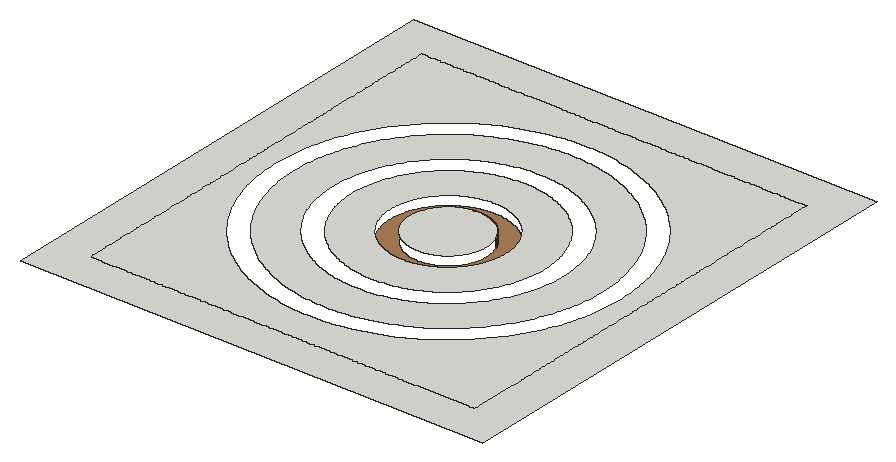
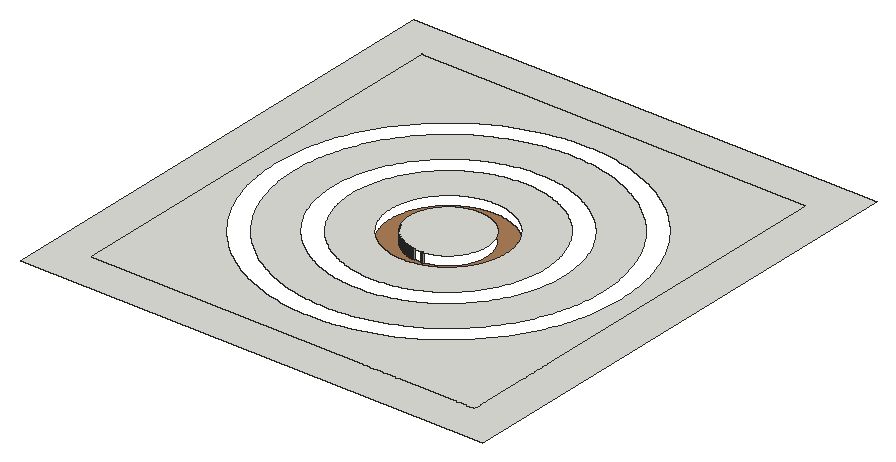
# SketchUp Ruby script. Lengths in inches.
U = 1.inch
M = Sketchup.active_model
def pt(a) = Geom::Point3d.new(a.map { |v| v * U })
def face(e, loops, mat)
  f = e.add_face(loops[0].map { |a| pt(a) })
  loops[1..].each { |l| e.add_face(l.map { |a| pt(a) }).erase! }
  f.material = f.back_material = mat if mat
  f
end
# faces: each face lists its corners as indices into pts; further lists are holes
def faces(e, pts, list, mat = nil) = list.each { |f| face(e, (f[0].is_a?(Array) ? f : [f]).map { |l| l.map { |i| pts[i] } }, mat) }
# xy, xz, yz: faces in a plane at the given z, y or x. An outline is a flat list of corners, or four numbers for a rectangle; further outlines are holes
def ring(l) = l.size == 4 ? [[l[0], l[1]], [l[2], l[1]], [l[2], l[3]], [l[0], l[3]]] : l.each_slice(2).to_a
def flat(e, list, mat, &to3) = list.each { |f| face(e, (f[0].is_a?(Array) ? f : [f]).map { |l| ring(l).map { |u, v| to3.(u, v) } }, mat) }
def xy(e, z, list, mat = nil) = flat(e, list, mat) { |x, y| [x, y, z] }
def xz(e, y, list, mat = nil) = flat(e, list, mat) { |x, z| [x, y, z] }
def yz(e, x, list, mat = nil) = flat(e, list, mat) { |y, z| [x, y, z] }
def lines(e, pts, list) = list.each { |a, b| e.add_line(pt(pts[a]), pt(pts[b])) }
# prism: a flat outline (further loops are holes) pulled along v
def prism(e, loops, v, mat = nil)
  f = face(e, loops, mat); d = Geom::Vector3d.new(v.map { |x| x * U })
  f.pushpull(f.normal.samedirection?(d) ? d.length : -d.length)
end
def box(e, o, s, mat = nil) = prism(e, [[o, [o[0] + s[0], o[1], o[2]], [o[0] + s[0], o[1] + s[1], o[2]], [o[0], o[1] + s[1], o[2]]]], [0, 0, s[2]], mat)
def at(x, y, z, deg = 0) = Geom::Transformation.translation(pt([x, y, z])) * Geom::Transformation.rotation(ORIGIN, Z_AXIS, deg.degrees)
def axes(o, x, y, z) = Geom::Transformation.new([*x, 0, *y, 0, *z, 0, *pt(o).to_a, 1])
def part(name) = M.definitions.add(name)
# library, detail: a bought-in or finely detailed component or shape, given as its bounding box
def library(name, o, s) = part(name).tap { |d| box(d.entities, o, s) }
def detail(e, o, s) = box(e.add_group.entities, o, s)
def put(e, d, t, mat = nil) = e.add_instance(d, t).tap { |i| i.material = mat if mat }
def group(e, t, mat = nil) = e.add_group.tap { |g| g.transformation = t; g.material = mat if mat }.entities
root = M.entities
M.materials.add("01 - Default1").color = [173, 128, 89]
xy(root,111.3125,[[[905.98,289.26,905.04,289.27,904.09,289.31,903.15,289.37,902.22,289.45,901.28,289.5625,900.35,289.7,899.42,289.86,898.49,290.04,897.57,290.25,896.66,290.48,895.75,290.74,894.85,291.02,893.96,291.32,893.08,291.65,892.2,292,891.34,292.37,890.48,292.76,889.64,293.18,888.8,293.62,887.98,294.08,887.17,294.5625,886.37,295.0625,885.59,295.59,884.82,296.13,884.0625,296.7,883.32,297.28,882.6,297.88,881.89,298.5,881.2,299.14,880.52,299.8,879.87,300.48,879.23,301.17,878.6,301.875,878,302.6,877.42,303.34,876.85,304.1,876.31,304.87,875.79,305.65,875.28,306.45,874.8,307.26,874.34,308.08,873.9,308.91,873.49,309.76,873.09,310.61,872.72,311.48,872.37,312.35,872.04,313.24,871.74,314.13,871.46,315.03,871.21,315.9375,870.97,316.85,870.77,317.77,870.58,318.7,870.42,319.625,870.29,320.56,870.18,321.49,870.09,322.43,870.03,323.37,869.99,324.3125,869.98,325.26,869.99,326.2,870.03,327.14,870.09,328.08,870.18,329.02,870.29,329.96,870.42,330.89,870.58,331.82,870.77,332.74,870.97,333.66,871.21,334.57,871.46,335.48,871.74,336.38,872.04,337.27,872.37,338.16,872.72,339.03,873.09,339.9,873.49,340.75,873.9,341.6,874.34,342.43,874.8,343.26,875.28,344.07,875.79,344.86,876.31,345.65,876.85,346.42,877.42,347.17,878,347.91,878.6,348.64,879.23,349.34,879.87,350.04,880.52,350.71,881.2,351.37,881.89,352.01,882.6,352.63,883.32,353.23,884.0625,353.82,884.82,354.38,885.59,354.92,886.37,355.45,887.17,355.95,887.98,356.43,888.8,356.89,889.64,357.33,890.48,357.75,891.34,358.14,892.2,358.52,893.08,358.87,893.96,359.19,894.85,359.49,895.75,359.77,896.66,360.03,897.57,360.26,898.49,360.47,899.42,360.65,900.35,360.8125,901.28,360.95,902.22,361.06,903.15,361.15,904.09,361.21,905.04,361.24,905.98,361.26,906.92,361.24,907.86,361.21,908.8,361.15,909.74,361.06,910.68,360.95,911.61,360.8125,912.54,360.65,913.46,360.47,914.38,360.26,915.3,360.03,916.2,359.77,917.1,359.49,918,359.19,918.88,358.87,919.76,358.52,920.62,358.14,921.48,357.75,922.32,357.33,923.16,356.89,923.98,356.43,924.79,355.95,925.59,355.45,926.37,354.92,927.14,354.38,927.89,353.82,928.63,353.23,929.36,352.63,930.07,352.01,930.76,351.37,931.43,350.71,932.09,350.04,932.73,349.34,933.35,348.64,933.96,347.91,934.54,347.17,935.1,346.42,935.65,345.65,936.17,344.86,936.67,344.07,937.16,343.26,937.62,342.43,938.05,341.6,938.47,340.75,938.87,339.9,939.24,339.03,939.59,338.16,939.91,337.27,940.22,336.38,940.5,335.48,940.75,334.57,940.98,333.66,941.19,332.74,941.375,331.82,941.54,330.89,941.67,329.96,941.78,329.02,941.87,328.08,941.93,327.14,941.97,326.2,941.98,325.26,941.97,324.3125,941.93,323.37,941.87,322.43,941.78,321.49,941.67,320.56,941.54,319.625,941.375,318.7,941.19,317.77,940.98,316.85,940.75,315.9375,940.5,315.03,940.22,314.13,939.91,313.24,939.59,312.35,939.24,311.48,938.87,310.61,938.47,309.76,938.05,308.91,937.62,308.08,937.16,307.26,936.67,306.45,936.17,305.65,935.65,304.87,935.1,304.1,934.54,303.34,933.96,302.6,933.35,301.875,932.73,301.17,932.09,300.48,931.43,299.8,930.76,299.14,930.07,298.5,929.36,297.88,928.63,297.28,927.89,296.7,927.14,296.13,926.37,295.59,925.59,295.0625,924.79,294.5625,923.98,294.08,923.16,293.62,922.32,293.18,921.48,292.76,920.62,292.37,919.76,292,918.88,291.65,918,291.32,917.1,291.02,916.2,290.74,915.3,290.48,914.38,290.25,913.46,290.04,912.54,289.86,911.61,289.7,910.68,289.5625,909.74,289.45,908.8,289.37,907.86,289.31,906.92,289.27],[905.35,301.26,906.61,301.26,907.23,301.29,907.86,301.33,908.49,301.39,909.11,301.46,909.73,301.55,910.35,301.66,910.97,301.78,911.58,301.92,912.19,302.07,912.8,302.24,913.4,302.43,913.99,302.63,914.58,302.85,915.16,303.08,915.74,303.33,916.3125,303.59,916.875,303.87,917.43,304.16,917.98,304.47,918.52,304.79,919.05,305.13,919.57,305.48,920.09,305.84,920.59,306.22,921.08,306.6,921.57,307.01,922.04,307.42,922.5,307.85,922.95,308.29,923.39,308.74,923.8125,309.2,924.23,309.67,924.63,310.15,925.02,310.65,925.4,311.15,925.76,311.66,926.11,312.18,926.44,312.72,926.76,313.26,927.07,313.8,927.36,314.36,927.64,314.92,927.9,315.49,928.15,316.07,928.38,316.66,928.6,317.24,928.8,317.84,928.99,318.44,929.16,319.04,929.32,319.65,929.45,320.27,929.58,320.88,929.68,321.5,929.77,322.125,929.85,322.75,929.95,324,929.97,324.63,929.98,325.26,929.97,325.88,929.95,326.51,929.9,327.14,929.85,327.76,929.77,328.39,929.68,329.01,929.58,329.63,929.45,330.25,929.32,330.86,929.16,331.47,928.99,332.07,928.8,332.67,928.6,333.27,928.38,333.86,928.15,334.44,927.9,335.02,927.64,335.59,927.36,336.15,927.07,336.71,926.76,337.26,926.44,337.8,926.11,338.33,925.76,338.85,925.4,339.36,925.02,339.87,924.63,340.36,924.23,340.84,923.8125,341.32,923.39,341.78,922.95,342.23,922.5,342.67,922.04,343.09,921.57,343.51,921.08,343.91,920.59,344.3,920.09,344.67,919.57,345.04,919.05,345.38,918.52,345.72,917.98,346.04,917.43,346.35,916.875,346.64,916.3125,346.92,915.74,347.18,915.16,347.43,914.58,347.66,913.99,347.88,913.4,348.08,912.8,348.27,912.19,348.4375,911.58,348.59,910.97,348.73,910.35,348.85,909.73,348.96,909.11,349.05,908.49,349.125,907.86,349.18,907.23,349.22,906.61,349.25,905.98,349.26,905.35,349.25,904.72,349.22,904.1,349.18,903.47,349.125,902.85,349.05,902.22,348.96,901.61,348.85,900.99,348.73,900.375,348.59,899.77,348.4375,899.16,348.27,898.5625,348.08,897.97,347.88,897.38,347.66,896.79,347.43,896.22,347.18,895.65,346.92,895.08,346.64,894.53,346.35,893.98,346.04,893.4375,345.72,892.91,345.38,892.38,345.04,891.87,344.67,891.37,344.3,890.875,343.91,890.39,343.51,889.92,343.09,889.46,342.67,889.01,342.23,888.57,341.78,888.14,341.32,887.73,340.84,887.33,340.36,886.9375,339.87,886.5625,339.36,886.2,338.85,885.85,338.33,885.52,337.8,885.19,337.26,884.89,336.71,884.59,336.15,884.32,335.59,884.05,335.02,883.57,333.86,883.36,333.27,883.15,332.67,882.97,332.07,882.8,331.47,882.64,330.86,882.5,330.25,882.38,329.63,882.27,329.01,882.18,328.39,882.11,327.76,882.05,327.14,882.01,326.51,881.99,325.88,881.98,325.26,881.99,324.63,882.01,324,882.05,323.375,882.11,322.75,882.18,322.125,882.27,321.5,882.38,320.88,882.5,320.27,882.64,319.65,882.8,319.04,882.97,318.44,883.15,317.84,883.36,317.24,883.57,316.66,883.81,316.07,884.05,315.49,884.32,314.92,884.59,314.36,884.89,313.8,885.19,313.26,885.85,312.18,886.2,311.66,886.5625,311.15,886.9375,310.65,887.33,310.15,887.73,309.67,888.14,309.2,888.57,308.74,889.01,308.29,889.46,307.85,889.92,307.42,890.39,307.01,890.875,306.6,891.37,306.22,891.87,305.84,892.38,305.48,892.91,305.13,893.4375,304.79,893.98,304.47,894.53,304.16,895.08,303.87,895.65,303.59,896.22,303.33,896.79,303.08,897.38,302.85,897.97,302.63,898.5625,302.43,899.16,302.24,899.77,302.07,900.375,301.92,900.99,301.78,901.61,301.66,902.22,301.55,902.85,301.46,903.47,301.39,904.1,301.33,904.72,301.29]]],"01 - Default1")
xy(root,117.3125,[[[761.98,172.26,1049.98,478.26],[785.98,196.26,1025.98,454.26]],[[785.98,196.26,1025.98,454.26],[905.89,217.26,908.71,217.29,911.54,217.4,914.36,217.58,917.18,217.84,919.98,218.17,922.78,218.57,925.57,219.05,928.34,219.6,931.1,220.22,933.84,220.91,936.5625,221.68,939.26,222.51,941.94,223.42,944.6,224.4,947.22,225.44,949.82,226.56,952.39,227.74,954.93,228.99,957.43,230.3,959.9,231.68,962.33,233.12,964.72,234.63,967.07,236.2,969.38,237.83,971.65,239.52,973.87,241.27,976.05,243.07,978.18,244.93,980.25,246.85,982.28,248.82,984.25,250.85,986.18,252.92,988.04,255.05,989.85,257.22,991.6,259.4375,993.3,261.7,994.93,264.01,996.5,266.36,998.02,268.75,999.46,271.18,1000.85,273.64,1002.17,276.14,1003.42,278.68,1004.6,281.24,1005.72,283.84,1006.77,286.47,1007.75,289.12,1008.66,291.79,1009.5,294.49,1010.27,297.21,1010.97,299.95,1011.6,302.71,1012.15,305.48,1012.63,308.27,1013.04,311.07,1013.38,313.875,1013.64,316.69,1013.83,319.51,1013.9375,322.34,1013.98,325.16,1013.94,327.99,1013.84,330.82,1013.65,333.64,1013.4,336.45,1013.07,339.26,1012.66,342.06,1012.1875,344.85,1011.64,347.62,1011.02,350.38,1010.32,353.12,1009.56,355.84,1008.72,358.54,1007.82,361.22,1006.84,363.87,1005.79,366.5,1004.68,369.1,1003.5,371.67,1002.25,374.2,1000.94,376.71,999.56,379.18,998.11,381.61,996.61,384,995.04,386.35,993.41,388.66,991.72,390.93,989.97,393.15,988.16,395.33,986.3,397.45,984.38,399.53,982.41,401.56,980.39,403.53,978.3125,405.45,976.19,407.32,974.02,409.13,971.8,410.88,969.53,412.58,967.23,414.21,964.88,415.78,962.49,417.29,960.06,418.74,957.59,420.125,955.09,421.44,952.56,422.7,949.99,423.88,947.39,425,944.77,426.05,942.12,427.03,939.44,427.94,936.74,428.78,934.02,429.55,931.28,430.25,928.52,430.875,925.75,431.43,922.97,431.91,920.17,432.32,917.36,432.65,914.55,432.92,911.72,433.1,908.9,433.22,906.07,433.26,903.24,433.22,900.42,433.11,897.6,432.93,894.78,432.67,891.97,432.34,889.18,431.94,886.39,431.46,883.62,430.92,880.86,430.29,878.12,429.6,875.39,428.84,872.69,428,870.02,427.09,867.36,426.12,864.74,425.07,862.14,423.96,859.57,422.78,857.03,421.53,854.53,420.21,852.06,418.83,849.63,417.39,847.24,415.88,844.88,414.31,842.57,412.68,840.31,411,838.08,409.25,835.91,407.44,833.78,405.58,831.7,403.66,829.68,401.69,827.7,399.67,825.78,397.59,823.92,395.47,822.11,393.3,820.35,391.08,818.66,388.8125,817.03,386.5,815.45,384.16,813.94,381.77,812.49,379.34,811.11,376.87,809.79,374.37,808.54,371.84,807.35,369.27,806.24,366.67,805.19,364.05,804.2,361.4,803.29,358.72,802.45,356.02,801.68,353.3,800.98,350.56,800.36,347.8,799.8,345.03,799.32,342.24,798.91,339.45,798.58,336.64,798.32,333.82,798.13,331,798.02,328.18,797.98,325.35,798.01,322.52,798.12,319.7,798.3,316.875,798.5625,314.06,798.89,311.25,799.29,308.45,799.77,305.67,800.32,302.89,800.94,300.13,801.63,297.39,802.4,294.67,803.24,291.97,804.14,289.29,805.12,286.64,806.16,284.01,807.28,281.41,808.46,278.85,809.71,276.31,811.02,273.81,812.4,271.34,813.84,268.91,815.35,266.51,816.92,264.16,818.55,261.85,820.24,259.58,821.99,257.36,823.79,255.1875,825.66,253.06,827.57,250.98,829.55,248.95,831.57,246.98,833.64,245.06,835.77,243.19,837.94,241.38,840.16,239.63,842.42,237.9375,844.73,236.3,847.08,234.73,849.47,233.22,851.9,231.77,854.36,230.39,856.86,229.07,859.4,227.82,861.97,226.63,864.5625,225.51,867.1875,224.46,869.84,223.48,872.52,222.57,875.22,221.73,877.9375,220.96,880.68,220.26,883.43,219.64,886.21,219.08,888.99,218.6,891.79,218.19,894.6,217.86,897.41,217.6,900.23,217.41,903.06,217.3]],[[905.98,229.26,903.47,229.29,900.95,229.39,898.45,229.55,895.94,229.78,893.45,230.08,890.96,230.4375,888.48,230.86,886.02,231.35,883.57,231.91,881.13,232.53,878.71,233.21,876.3125,233.95,873.93,234.76,871.58,235.63,869.24,236.5625,866.93,237.56,864.65,238.61,862.4,239.72,860.17,240.89,857.98,242.12,855.82,243.4,853.69,244.74,851.6,246.14,849.55,247.59,847.54,249.09,845.5625,250.65,843.63,252.26,841.74,253.91,839.9,255.62,838.1,257.375,836.34,259.17,834.64,261.02,832.98,262.91,831.37,264.84,829.82,266.82,828.3125,268.83,826.86,270.88,825.47,272.97,824.125,275.1,822.84,277.26,821.61,279.45,820.44,281.67,819.33,283.93,818.28,286.21,817.29,288.52,816.35,290.85,815.49,293.21,814.68,295.59,813.93,297.99,813.25,300.41,812.63,302.85,812.08,305.3,811.59,307.76,811.16,310.24,810.8,312.73,810.5,315.22,810.27,317.72,810.11,320.23,810.01,322.74,809.98,325.26,810.01,327.77,810.11,330.28,810.27,332.79,810.5,335.29,810.8,337.79,811.16,340.27,811.59,342.75,812.08,345.22,812.63,347.67,813.25,350.1,813.93,352.52,814.68,354.92,815.49,357.3,816.35,359.66,817.29,361.99,818.28,364.3,819.33,366.59,820.44,368.84,821.61,371.0625,822.84,373.26,824.125,375.42,825.47,377.54,826.86,379.63,828.3125,381.68,829.82,383.7,831.37,385.67,832.98,387.6,834.64,389.49,836.34,391.34,838.1,393.14,839.9,394.89,841.74,396.6,843.63,398.26,845.5625,399.86,847.54,401.42,849.55,402.92,851.6,404.37,853.69,405.77,855.82,407.11,857.98,408.39,860.17,409.62,862.4,410.79,864.65,411.9,866.93,412.96,869.24,413.95,871.58,414.88,873.93,415.75,876.3125,416.56,878.71,417.3,881.13,417.99,883.57,418.6,886.02,419.16,888.48,419.65,890.96,420.07,893.45,420.43,895.94,420.73,898.45,420.96,900.95,421.125,903.47,421.22,905.98,421.26,908.49,421.22,911,421.125,913.51,420.96,916.01,420.73,918.51,420.43,921,420.07,923.47,419.65,925.9375,419.16,928.39,418.6,930.83,417.99,933.24,417.3,935.64,416.56,938.02,415.75,940.38,414.88,942.72,413.95,945.03,412.96,947.31,411.9,949.5625,410.79,951.79,409.62,953.98,408.39,956.14,407.11,958.26,405.77,960.35,404.37,962.41,402.92,964.42,401.42,966.39,399.86,968.33,398.26,970.22,396.6,972.0625,394.89,973.86,393.14,975.61,391.34,977.32,389.49,978.98,387.6,980.58,385.67,982.14,383.7,983.64,381.68,985.09,379.63,986.49,377.54,987.83,375.42,989.12,373.26,990.35,371.0625,991.52,368.84,992.625,366.59,993.68,364.3,994.67,361.99,995.6,359.66,996.47,357.3,997.28,354.92,998.03,352.52,998.71,350.1,999.33,347.67,999.88,345.22,1000.37,342.75,1000.8,340.27,1001.16,337.79,1001.45,335.29,1001.68,332.79,1001.85,330.28,1001.95,327.77,1001.98,325.26,1001.95,322.74,1001.85,320.23,1001.68,317.72,1001.45,315.22,1001.16,312.73,1000.8,310.24,1000.37,307.76,999.88,305.3,999.33,302.85,998.71,300.41,998.03,297.99,997.28,295.59,996.47,293.21,995.6,290.85,994.67,288.52,993.68,286.21,992.625,283.93,991.52,281.67,990.35,279.45,989.12,277.26,987.83,275.1,986.49,272.97,985.09,270.88,983.64,268.83,982.14,266.82,980.58,264.84,978.98,262.91,977.32,261.02,975.61,259.17,973.86,257.375,972.0625,255.62,970.22,253.91,968.33,252.26,966.39,250.65,964.42,249.09,962.41,247.59,960.35,246.14,958.26,244.74,956.14,243.4,953.98,242.12,951.79,240.89,949.5625,239.72,947.31,238.61,945.03,237.56,942.72,236.5625,940.38,235.63,938.02,234.76,935.64,233.95,933.24,233.21,930.83,232.53,928.39,231.91,925.9375,231.35,923.47,230.86,921,230.4375,918.51,230.08,916.01,229.78,913.51,229.55,911,229.39,908.49,229.29],[905.98,253.26,907.86,253.28,909.75,253.35,911.63,253.48,913.5,253.65,915.375,253.87,917.24,254.14,919.1,254.46,920.95,254.83,922.79,255.25,924.61,255.71,926.43,256.22,928.23,256.78,930.01,257.39,931.78,258.04,933.53,258.74,935.26,259.48,936.98,260.27,938.67,261.1,940.33,261.98,941.98,262.9,943.6,263.87,945.19,264.87,946.76,265.92,948.3,267.01,949.81,268.13,951.29,269.3,952.74,270.51,954.16,271.75,955.54,273.03,956.89,274.34,958.21,275.69,959.49,277.08,960.73,278.5,961.93,279.95,963.1,281.43,964.23,282.9375,965.32,284.47,966.36,286.04,967.37,287.64,968.33,289.26,969.25,290.9,970.13,292.57,970.96,294.26,971.75,295.97,972.5,297.7,973.2,299.45,973.85,301.22,974.45,303.01,975.01,304.81,975.53,306.62,975.99,308.45,976.41,310.29,976.77,312.14,977.09,313.99,977.36,315.86,977.58,317.73,977.76,319.61,977.88,321.49,977.95,323.37,977.98,325.26,977.95,327.14,977.88,329.02,977.76,330.91,977.58,332.78,977.36,334.65,977.09,336.52,976.77,338.38,976.41,340.23,975.99,342.0625,975.53,343.89,975.01,345.71,974.45,347.51,973.85,349.29,973.2,351.06,972.5,352.81,971.75,354.54,970.96,356.25,970.13,357.94,969.25,359.61,968.33,361.26,967.37,362.875,966.36,364.47,965.32,366.04,964.23,367.58,963.1,369.09,961.93,370.57,960.73,372.02,959.49,373.43,958.21,374.82,956.89,376.17,955.54,377.48,954.16,378.76,952.74,380.01,951.29,381.21,949.81,382.38,948.3,383.51,946.76,384.59,945.19,385.64,943.6,386.65,941.98,387.61,940.33,388.53,938.67,389.41,936.98,390.24,935.26,391.03,933.53,391.78,931.78,392.47,930.01,393.125,928.23,393.73,926.43,394.29,924.61,394.8,922.79,395.27,920.95,395.68,919.1,396.05,917.24,396.37,915.375,396.64,913.5,396.86,911.63,397.03,909.75,397.16,907.86,397.23,905.98,397.26,904.09,397.23,902.21,397.16,900.33,397.03,898.45,396.86,896.58,396.64,894.72,396.37,892.86,396.05,891.01,395.68,889.17,395.27,887.34,394.8,885.53,394.29,883.73,393.73,881.94,393.125,880.18,392.47,878.43,391.78,876.69,391.03,874.98,390.24,873.29,389.41,871.625,388.53,869.98,387.61,868.36,386.65,866.76,385.64,865.2,384.59,863.66,383.51,862.15,382.38,860.67,381.21,859.22,380.01,857.8,378.76,856.42,377.48,855.07,376.17,853.75,374.82,852.47,373.43,851.23,372.02,850.02,370.57,848.86,369.09,847.73,367.58,846.64,366.04,845.59,364.47,844.59,362.875,843.625,361.26,842.7,359.61,841.83,357.94,840.99,356.25,840.2,354.54,839.46,352.81,838.76,351.06,838.11,349.29,837.5,347.51,836.94,345.71,836.43,343.89,835.97,342.0625,835.55,340.23,835.18,338.38,834.87,336.52,834.59,334.65,834.375,332.78,834.2,330.91,834.08,329.02,834,327.14,833.98,325.26,834,323.37,834.08,321.49,834.2,319.61,834.375,317.73,834.59,315.86,834.87,313.99,835.18,312.14,835.55,310.29,835.97,308.45,836.43,306.62,836.94,304.81,837.5,303.01,838.11,301.22,838.76,299.45,839.46,297.7,840.2,295.97,840.99,294.26,841.83,292.57,842.7,290.9,843.625,289.26,844.59,287.64,845.59,286.04,846.64,284.47,847.73,282.9375,848.86,281.43,850.02,279.95,851.23,278.5,852.47,277.08,853.75,275.69,855.07,274.34,856.42,273.03,857.8,271.75,859.22,270.51,860.67,269.3,862.15,268.13,863.66,267.01,865.2,265.92,866.76,264.87,868.36,263.87,869.98,262.9,871.625,261.98,873.29,261.1,874.98,260.27,876.69,259.48,878.43,258.74,880.18,258.04,881.94,257.39,883.73,256.78,885.53,256.22,887.34,255.71,889.17,255.25,891.01,254.83,892.86,254.46,894.72,254.14,896.58,253.87,898.45,253.65,900.33,253.48,902.21,253.35,904.09,253.28]],[[905.98,265.26,904.41,265.28,902.84,265.34,901.27,265.44,899.71,265.58,898.15,265.77,896.59,265.99,895.04,266.26,893.5,266.57,891.97,266.91,890.45,267.3,888.9375,267.73,887.4375,268.19,885.95,268.7,884.48,269.24,883.02,269.82,881.57,270.44,880.15,271.1,878.74,271.8,877.35,272.53,875.98,273.29,874.63,274.1,873.3,274.9375,871.99,275.81,870.71,276.72,869.45,277.66,868.22,278.63,867.01,279.63,865.83,280.67,864.68,281.73,863.55,282.83,862.46,283.95,861.39,285.11,860.35,286.29,859.35,287.5,858.38,288.73,857.4375,289.99,856.53,291.27,855.66,292.58,854.82,293.91,854.02,295.26,853.25,296.625,852.52,298.02,851.82,299.43,851.17,300.85,850.55,302.3,849.96,303.75,849.42,305.23,848.92,306.72,848.45,308.22,848.02,309.73,847.64,311.25,847.29,312.78,846.98,314.32,846.72,315.87,846.49,317.42,846.31,318.98,846.16,320.55,846.0625,322.12,846,323.6875,845.98,325.26,846,326.83,846.0625,328.4,846.16,329.96,846.31,331.53,846.49,333.09,846.72,334.64,846.98,336.19,847.29,337.73,847.64,339.26,848.02,340.79,848.45,342.3,848.92,343.8,849.42,345.28,849.96,346.76,850.55,348.22,851.17,349.66,851.82,351.09,852.52,352.5,853.25,353.89,854.02,355.26,854.82,356.61,855.66,357.93,856.53,359.24,857.4375,360.52,858.38,361.78,859.35,363.02,860.35,364.22,861.39,365.4,862.46,366.56,863.55,367.68,864.68,368.78,865.83,369.84,867.01,370.88,868.22,371.88,869.45,372.86,870.71,373.8,871.99,374.7,873.3,375.58,874.63,376.41,875.98,377.22,877.35,377.99,878.74,378.72,880.15,379.41,881.57,380.07,883.02,380.6875,884.48,381.27,885.95,381.81,887.4375,382.32,888.9375,382.79,890.45,383.21,891.97,383.6,893.5,383.95,895.04,384.25,896.59,384.52,898.15,384.74,899.71,384.93,901.27,385.07,902.84,385.17,904.41,385.24,905.98,385.26,907.55,385.24,909.12,385.17,910.6875,385.07,912.25,384.93,913.81,384.74,915.36,384.52,916.91,384.25,918.45,383.95,919.99,383.6,921.51,383.21,923.02,382.79,924.52,382.32,926.01,381.81,927.48,381.27,928.94,380.6875,930.38,380.07,931.81,379.41,933.22,378.72,934.61,377.99,935.98,377.22,937.33,376.41,938.66,375.58,939.96,374.7,941.25,373.8,942.5,372.86,943.74,371.88,944.95,370.88,946.125,369.84,947.28,368.78,948.41,367.68,949.5,366.56,950.57,365.4,951.6,364.22,952.61,363.02,953.58,361.78,954.52,360.52,955.43,359.24,956.3,357.93,957.14,356.61,957.94,355.26,958.71,353.89,959.4375,352.5,960.13,351.09,960.79,349.66,961.41,348.22,961.99,346.76,962.54,345.28,963.04,343.8,963.51,342.3,963.93,340.79,964.32,339.26,964.67,337.73,964.97,336.19,965.24,334.64,965.47,333.09,965.65,331.53,965.79,329.96,965.9,328.4,965.96,326.83,965.98,325.26,965.96,323.6875,965.9,322.12,965.79,320.55,965.65,318.98,965.47,317.42,965.24,315.87,964.97,314.32,964.67,312.78,964.32,311.25,963.93,309.73,963.51,308.22,963.04,306.72,962.54,305.23,961.99,303.75,961.41,302.3,960.79,300.85,960.13,299.43,959.4375,298.02,958.71,296.625,957.94,295.26,957.14,293.91,956.3,292.58,955.43,291.27,954.52,289.99,953.58,288.73,952.61,287.5,951.6,286.29,950.57,285.11,949.5,283.95,948.41,282.83,947.28,281.73,946.125,280.67,944.95,279.63,943.74,278.63,942.5,277.66,941.25,276.72,939.96,275.81,938.66,274.9375,937.33,274.1,935.98,273.29,934.61,272.53,933.22,271.8,931.81,271.1,930.38,270.44,928.94,269.82,927.48,269.24,926.01,268.7,924.52,268.19,923.02,267.73,921.51,267.3,919.99,266.91,918.45,266.57,916.91,266.26,915.36,265.99,913.81,265.77,912.25,265.58,910.6875,265.44,909.12,265.34,907.55,265.28],[905.98,289.26,906.92,289.27,907.86,289.31,908.8,289.37,909.74,289.45,910.68,289.5625,911.61,289.7,912.54,289.86,913.46,290.04,914.38,290.25,915.3,290.48,916.2,290.74,917.1,291.02,918,291.32,918.88,291.65,919.76,292,920.62,292.37,921.48,292.76,922.32,293.18,923.16,293.62,923.98,294.08,924.79,294.5625,925.59,295.0625,926.37,295.59,927.14,296.13,927.89,296.7,928.63,297.28,929.36,297.88,930.07,298.5,930.76,299.14,931.43,299.8,932.09,300.48,932.73,301.17,933.35,301.875,933.96,302.6,934.54,303.34,935.1,304.1,935.65,304.87,936.17,305.65,936.67,306.45,937.16,307.26,937.62,308.08,938.05,308.91,938.47,309.76,938.87,310.61,939.24,311.48,939.59,312.35,939.91,313.24,940.22,314.13,940.5,315.03,940.75,315.9375,940.98,316.85,941.19,317.77,941.375,318.7,941.54,319.625,941.67,320.56,941.78,321.49,941.87,322.43,941.93,323.37,941.97,324.3125,941.98,325.26,941.97,326.2,941.93,327.14,941.87,328.08,941.78,329.02,941.67,329.96,941.54,330.89,941.375,331.82,941.19,332.74,940.98,333.66,940.75,334.57,940.5,335.48,940.22,336.38,939.91,337.27,939.59,338.16,939.24,339.03,938.87,339.9,938.47,340.75,938.05,341.6,937.62,342.43,937.16,343.26,936.67,344.07,936.17,344.86,935.65,345.65,935.1,346.42,934.54,347.17,933.96,347.91,933.35,348.64,932.73,349.34,932.09,350.04,931.43,350.71,930.76,351.37,930.07,352.01,929.36,352.63,928.63,353.23,927.89,353.82,927.14,354.38,926.37,354.92,925.59,355.45,924.79,355.95,923.98,356.43,923.16,356.89,922.32,357.33,921.48,357.75,920.62,358.14,919.76,358.52,918.88,358.87,918,359.19,917.1,359.49,916.2,359.77,915.3,360.03,914.38,360.26,913.46,360.47,912.54,360.65,911.61,360.8125,910.68,360.95,909.74,361.06,908.8,361.15,907.86,361.21,906.92,361.24,905.98,361.26,905.04,361.24,904.09,361.21,903.15,361.15,902.22,361.06,901.28,360.95,900.35,360.8125,899.42,360.65,898.49,360.47,897.57,360.26,896.66,360.03,895.75,359.77,894.85,359.49,893.96,359.19,893.08,358.87,892.2,358.52,891.34,358.14,890.48,357.75,889.64,357.33,888.8,356.89,887.98,356.43,887.17,355.95,886.37,355.45,885.59,354.92,884.82,354.38,884.0625,353.82,883.32,353.23,882.6,352.63,881.89,352.01,881.2,351.37,880.52,350.71,879.87,350.04,879.23,349.34,878.6,348.64,878,347.91,877.42,347.17,876.85,346.42,876.31,345.65,875.79,344.86,875.28,344.07,874.8,343.26,874.34,342.43,873.9,341.6,873.49,340.75,873.09,339.9,872.72,339.03,872.37,338.16,872.04,337.27,871.74,336.38,871.46,335.48,871.21,334.57,870.97,333.66,870.77,332.74,870.58,331.82,870.42,330.89,870.29,329.96,870.18,329.02,870.09,328.08,870.03,327.14,869.99,326.2,869.98,325.26,869.99,324.3125,870.03,323.37,870.09,322.43,870.18,321.49,870.29,320.56,870.42,319.625,870.58,318.7,870.77,317.77,870.97,316.85,871.21,315.9375,871.46,315.03,871.74,314.13,872.04,313.24,872.37,312.35,872.72,311.48,873.09,310.61,873.49,309.76,873.9,308.91,874.34,308.08,874.8,307.26,875.28,306.45,875.79,305.65,876.31,304.87,876.85,304.1,877.42,303.34,878,302.6,878.6,301.875,879.23,301.17,879.87,300.48,880.52,299.8,881.2,299.14,881.89,298.5,882.6,297.88,883.32,297.28,884.0625,296.7,884.82,296.13,885.59,295.59,886.37,295.0625,887.17,294.5625,887.98,294.08,888.8,293.62,889.64,293.18,890.48,292.76,891.34,292.37,892.2,292,893.08,291.65,893.96,291.32,894.85,291.02,895.75,290.74,896.66,290.48,897.57,290.25,898.49,290.04,899.42,289.86,900.35,289.7,901.28,289.5625,902.22,289.45,903.15,289.37,904.09,289.31,905.04,289.27]],[905.35,301.26,904.72,301.29,904.1,301.33,903.47,301.39,902.85,301.46,902.22,301.55,901.61,301.66,900.99,301.78,900.375,301.92,899.77,302.07,899.16,302.24,898.5625,302.43,897.97,302.63,897.38,302.85,896.79,303.08,896.22,303.33,895.65,303.59,895.08,303.87,894.53,304.16,893.98,304.47,893.4375,304.79,892.91,305.13,892.38,305.48,891.87,305.84,891.37,306.22,890.875,306.6,890.39,307.01,889.92,307.42,889.46,307.85,889.01,308.29,888.57,308.74,888.14,309.2,887.73,309.67,887.33,310.15,886.9375,310.65,886.5625,311.15,886.2,311.66,885.85,312.18,885.19,313.26,884.89,313.8,884.59,314.36,884.32,314.92,884.05,315.49,883.81,316.07,883.57,316.66,883.36,317.24,883.15,317.84,882.97,318.44,882.8,319.04,882.64,319.65,882.5,320.27,882.38,320.88,882.27,321.5,882.18,322.125,882.11,322.75,882.05,323.375,882.01,324,881.99,324.63,881.98,325.26,881.99,325.88,882.01,326.51,882.05,327.14,882.11,327.76,882.18,328.39,882.27,329.01,882.38,329.63,882.5,330.25,882.64,330.86,882.8,331.47,882.97,332.07,883.15,332.67,883.36,333.27,883.57,333.86,884.05,335.02,884.32,335.59,884.59,336.15,884.89,336.71,885.19,337.26,885.52,337.8,885.85,338.33,886.2,338.85,886.5625,339.36,886.9375,339.87,887.33,340.36,887.73,340.84,888.14,341.32,888.57,341.78,889.01,342.23,889.46,342.67,889.92,343.09,890.39,343.51,890.875,343.91,891.37,344.3,891.87,344.67,892.38,345.04,892.91,345.38,893.4375,345.72,893.98,346.04,894.53,346.35,895.08,346.64,895.65,346.92,896.22,347.18,896.79,347.43,897.38,347.66,897.97,347.88,898.5625,348.08,899.16,348.27,899.77,348.4375,900.375,348.59,900.99,348.73,901.61,348.85,902.22,348.96,902.85,349.05,903.47,349.125,904.1,349.18,904.72,349.22,905.35,349.25,905.98,349.26,906.61,349.25,907.23,349.22,907.86,349.18,908.49,349.125,909.11,349.05,909.73,348.96,910.35,348.85,910.97,348.73,911.58,348.59,912.19,348.4375,912.8,348.27,913.4,348.08,913.99,347.88,914.58,347.66,915.16,347.43,915.74,347.18,916.3125,346.92,916.875,346.64,917.43,346.35,917.98,346.04,918.52,345.72,919.05,345.38,919.57,345.04,920.09,344.67,920.59,344.3,921.08,343.91,921.57,343.51,922.04,343.09,922.5,342.67,922.95,342.23,923.39,341.78,923.8125,341.32,924.23,340.84,924.63,340.36,925.02,339.87,925.4,339.36,925.76,338.85,926.11,338.33,926.44,337.8,926.76,337.26,927.07,336.71,927.36,336.15,927.64,335.59,927.9,335.02,928.15,334.44,928.38,333.86,928.6,333.27,928.8,332.67,928.99,332.07,929.16,331.47,929.32,330.86,929.45,330.25,929.58,329.63,929.68,329.01,929.77,328.39,929.85,327.76,929.9,327.14,929.95,326.51,929.97,325.88,929.98,325.26,929.97,324.63,929.95,324,929.85,322.75,929.77,322.125,929.68,321.5,929.58,320.88,929.45,320.27,929.32,319.65,929.16,319.04,928.99,318.44,928.8,317.84,928.6,317.24,928.38,316.66,928.15,316.07,927.9,315.49,927.64,314.92,927.36,314.36,927.07,313.8,926.76,313.26,926.44,312.72,926.11,312.18,925.76,311.66,925.4,311.15,925.02,310.65,924.63,310.15,924.23,309.67,923.8125,309.2,923.39,308.74,922.95,308.29,922.5,307.85,922.04,307.42,921.57,307.01,921.08,306.6,920.59,306.22,920.09,305.84,919.57,305.48,919.05,305.13,918.52,304.79,917.98,304.47,917.43,304.16,916.875,303.87,916.3125,303.59,915.74,303.33,915.16,303.08,914.58,302.85,913.99,302.63,913.4,302.43,912.8,302.24,912.19,302.07,911.58,301.92,910.97,301.78,910.35,301.66,909.73,301.55,909.11,301.46,908.49,301.39,907.86,301.33,907.23,301.29,906.61,301.26]])
p = [[927.9,335.02,117.3125],[927.64,335.59,117.3125],[927.64,335.59,111.3125],[927.9,335.02,111.3125],[927.36,336.15,117.3125],[927.36,336.15,111.3125],
  [927.07,336.71,117.3125],[927.07,336.71,111.3125],[926.76,337.26,117.3125],[926.76,337.26,111.3125],[926.44,337.8,117.3125],[926.44,337.8,111.3125],
  [926.11,338.33,117.3125],[926.11,338.33,111.3125],[925.76,338.85,117.3125],[925.76,338.85,111.3125],[925.4,339.36,117.3125],[925.4,339.36,111.3125],
  [925.02,339.87,117.3125],[925.02,339.87,111.3125],[924.63,340.36,117.3125],[924.63,340.36,111.3125],[924.23,340.84,117.3125],[924.23,340.84,111.3125],
  [923.8125,341.32,117.3125],[923.8125,341.32,111.3125],[923.39,341.78,117.3125],[923.39,341.78,111.3125],[922.95,342.23,117.3125],[922.95,342.23,111.3125],
  [922.5,342.67,117.3125],[922.5,342.67,111.3125],[922.04,343.09,117.3125],[922.04,343.09,111.3125],[921.57,343.51,117.3125],[921.57,343.51,111.3125],
  [921.08,343.91,117.3125],[921.08,343.91,111.3125],[920.59,344.3,117.3125],[920.59,344.3,111.3125],[920.09,344.67,117.3125],[920.09,344.67,111.3125],
  [919.57,345.04,117.3125],[919.57,345.04,111.3125],[919.05,345.38,117.3125],[919.05,345.38,111.3125],[918.52,345.72,117.3125],[918.52,345.72,111.3125],
  [917.98,346.04,117.3125],[917.98,346.04,111.3125],[917.43,346.35,117.3125],[917.43,346.35,111.3125],[916.875,346.64,117.3125],[916.875,346.64,111.3125],
  [916.3125,346.92,117.3125],[916.3125,346.92,111.3125],[915.74,347.18,117.3125],[915.74,347.18,111.3125],[915.16,347.43,117.3125],[915.16,347.43,111.3125],
  [914.58,347.66,117.3125],[914.58,347.66,111.3125],[913.99,347.88,117.3125],[913.99,347.88,111.3125],[913.4,348.08,117.3125],[913.4,348.08,111.3125],
  [912.8,348.27,117.3125],[912.8,348.27,111.3125],[912.19,348.4375,117.3125],[912.19,348.4375,111.3125],[911.58,348.59,117.3125],[911.58,348.59,111.3125],
  [910.97,348.73,117.3125],[910.97,348.73,111.3125],[910.35,348.85,117.3125],[910.35,348.85,111.3125],[909.73,348.96,117.3125],[909.73,348.96,111.3125],
  [902.85,349.05,117.3125],[902.22,348.96,117.3125],[902.22,348.96,111.3125],[902.85,349.05,111.3125],[909.11,349.05,117.3125],[909.11,349.05,111.3125],
  [903.47,349.125,117.3125],[903.47,349.125,111.3125],[904.1,349.18,117.3125],[904.1,349.18,111.3125],[908.49,349.125,117.3125],[907.86,349.18,117.3125],
  [907.86,349.18,111.3125],[908.49,349.125,111.3125]]
faces(root,p,[[0,1,2,3],[1,4,5,2],[4,6,7,5],[6,8,9,7],[8,10,11,9],[10,12,13,11],[12,14,15,13],[14,16,17,15],
  [16,18,19,17],[18,20,21,19],[20,22,23,21],[22,24,25,23],[24,26,27,25],[26,28,29,27],[28,30,31,29],[30,32,33,31],
  [32,34,35,33],[34,36,37,35],[36,38,39,37],[38,40,41,39],[40,42,43,41],[42,44,45,43],[44,46,47,45],[46,48,49,47],
  [48,50,51,49],[50,52,53,51],[52,54,55,53],[54,56,57,55],[56,58,59,57],[58,60,61,59],[60,62,63,61],[62,64,65,63],
  [64,66,67,65],[66,68,69,67],[68,70,71,69],[70,72,73,71],[72,74,75,73],[74,76,77,75],[78,79,80,81],[76,82,83,77],
  [84,78,81,85],[86,84,85,87],[88,89,90,91],[82,88,91,83]])
